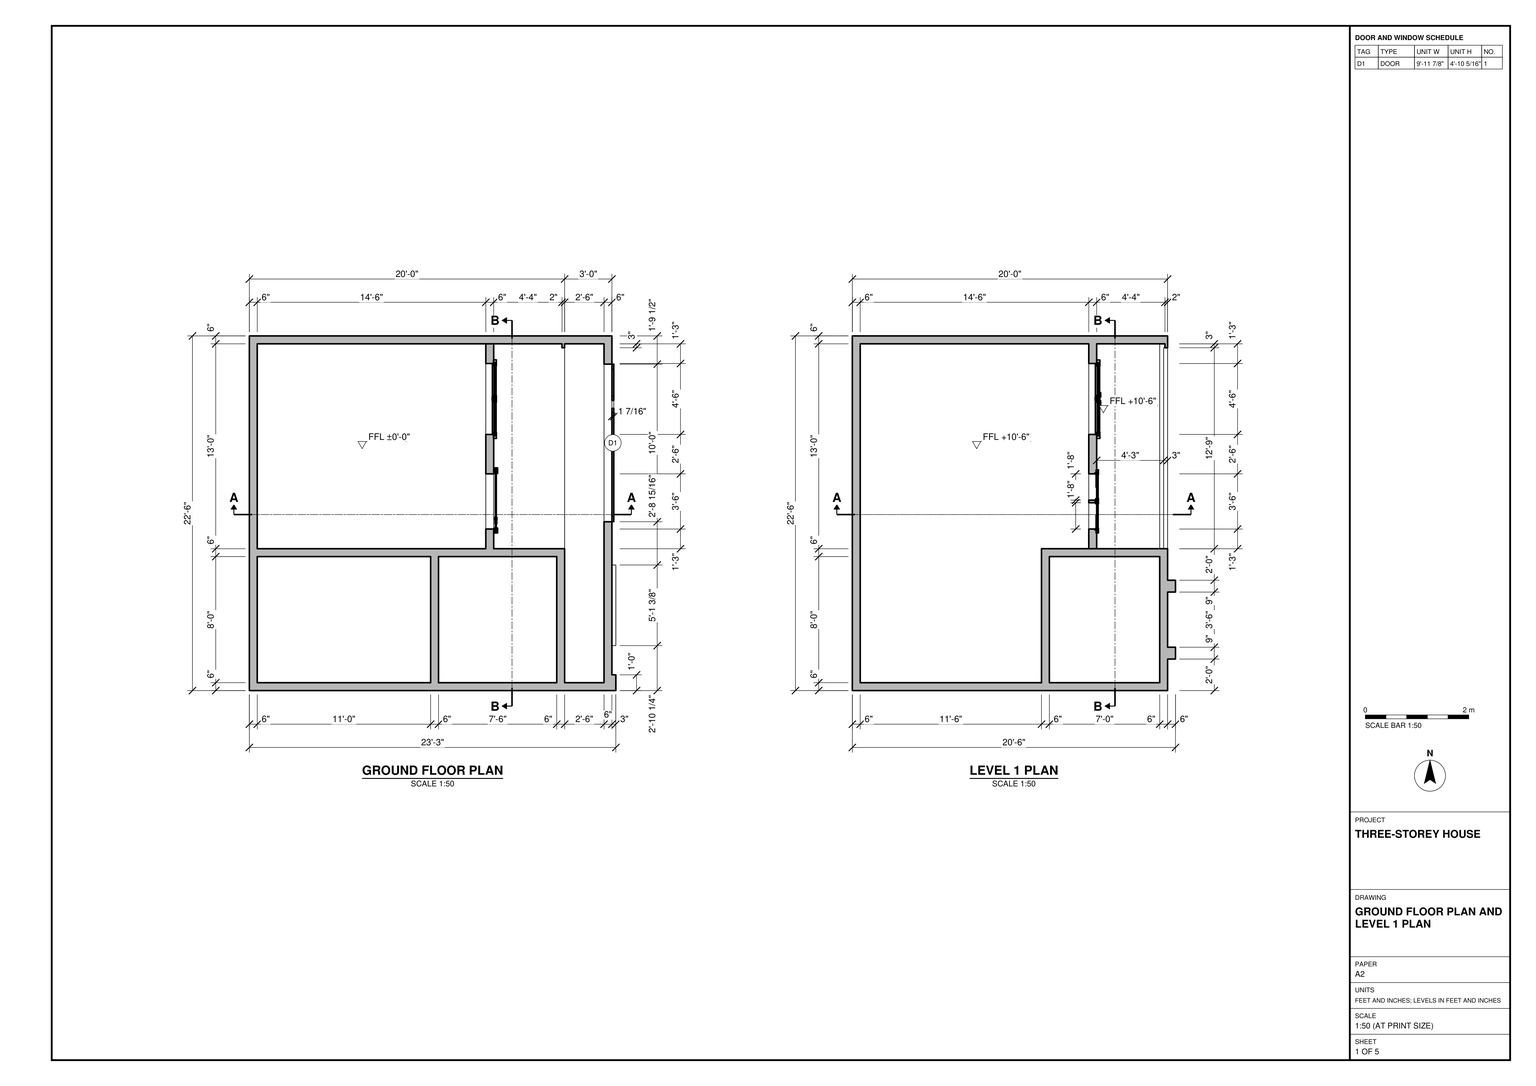
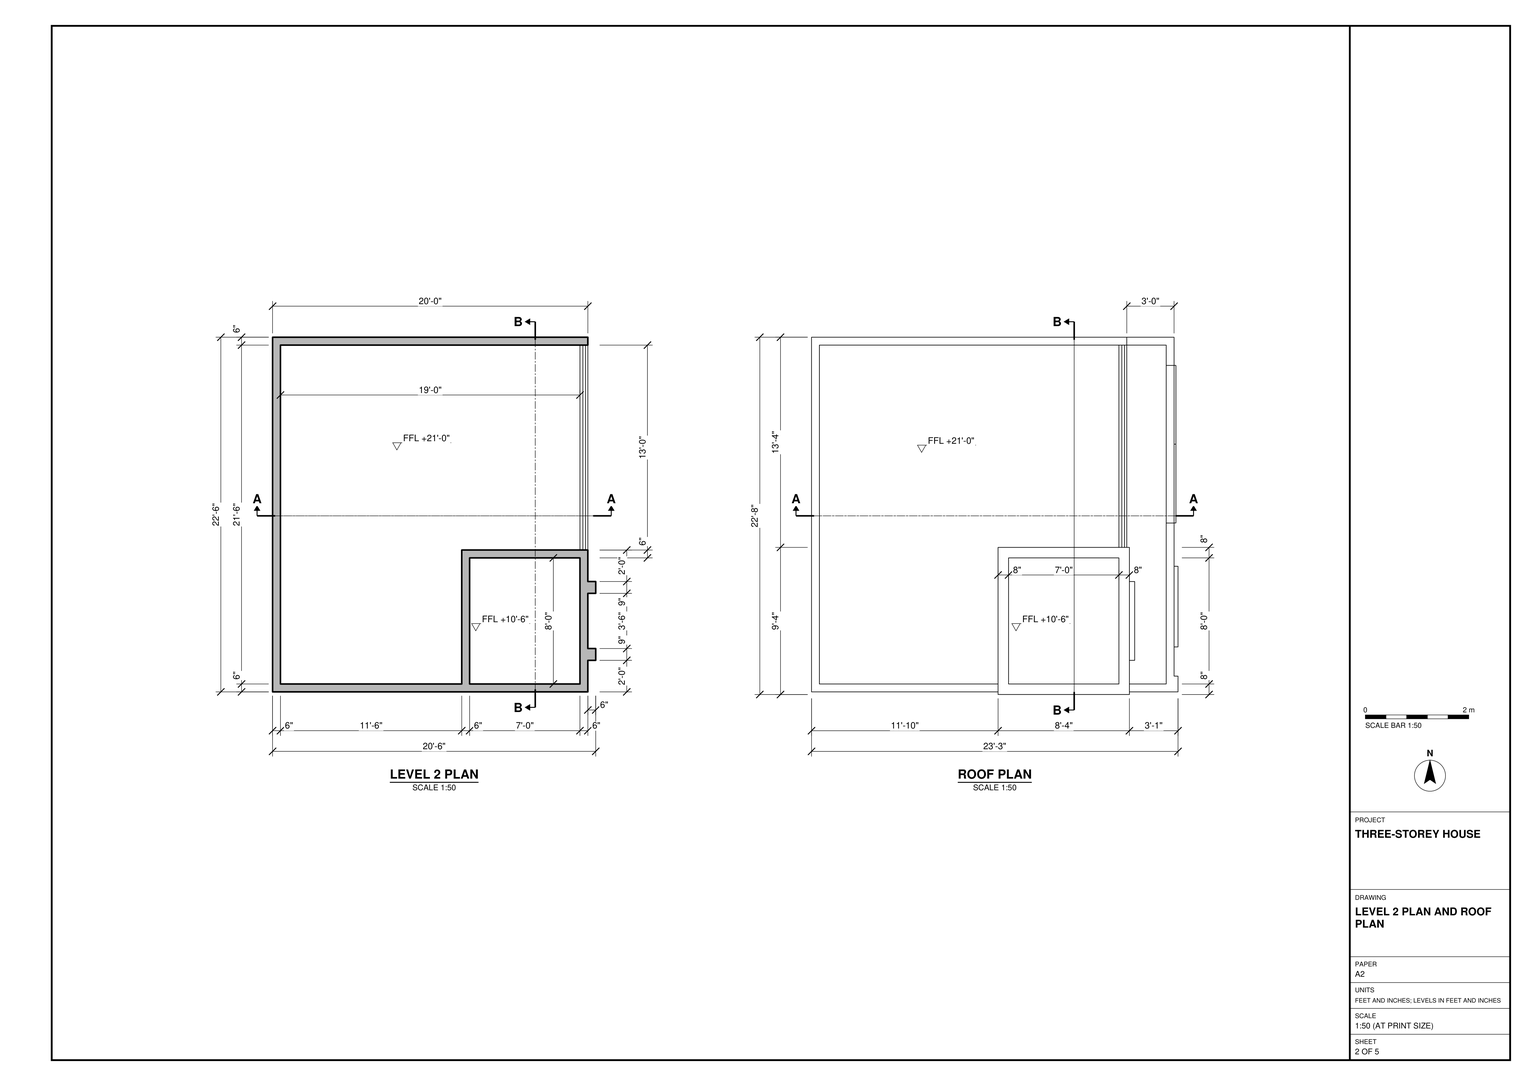
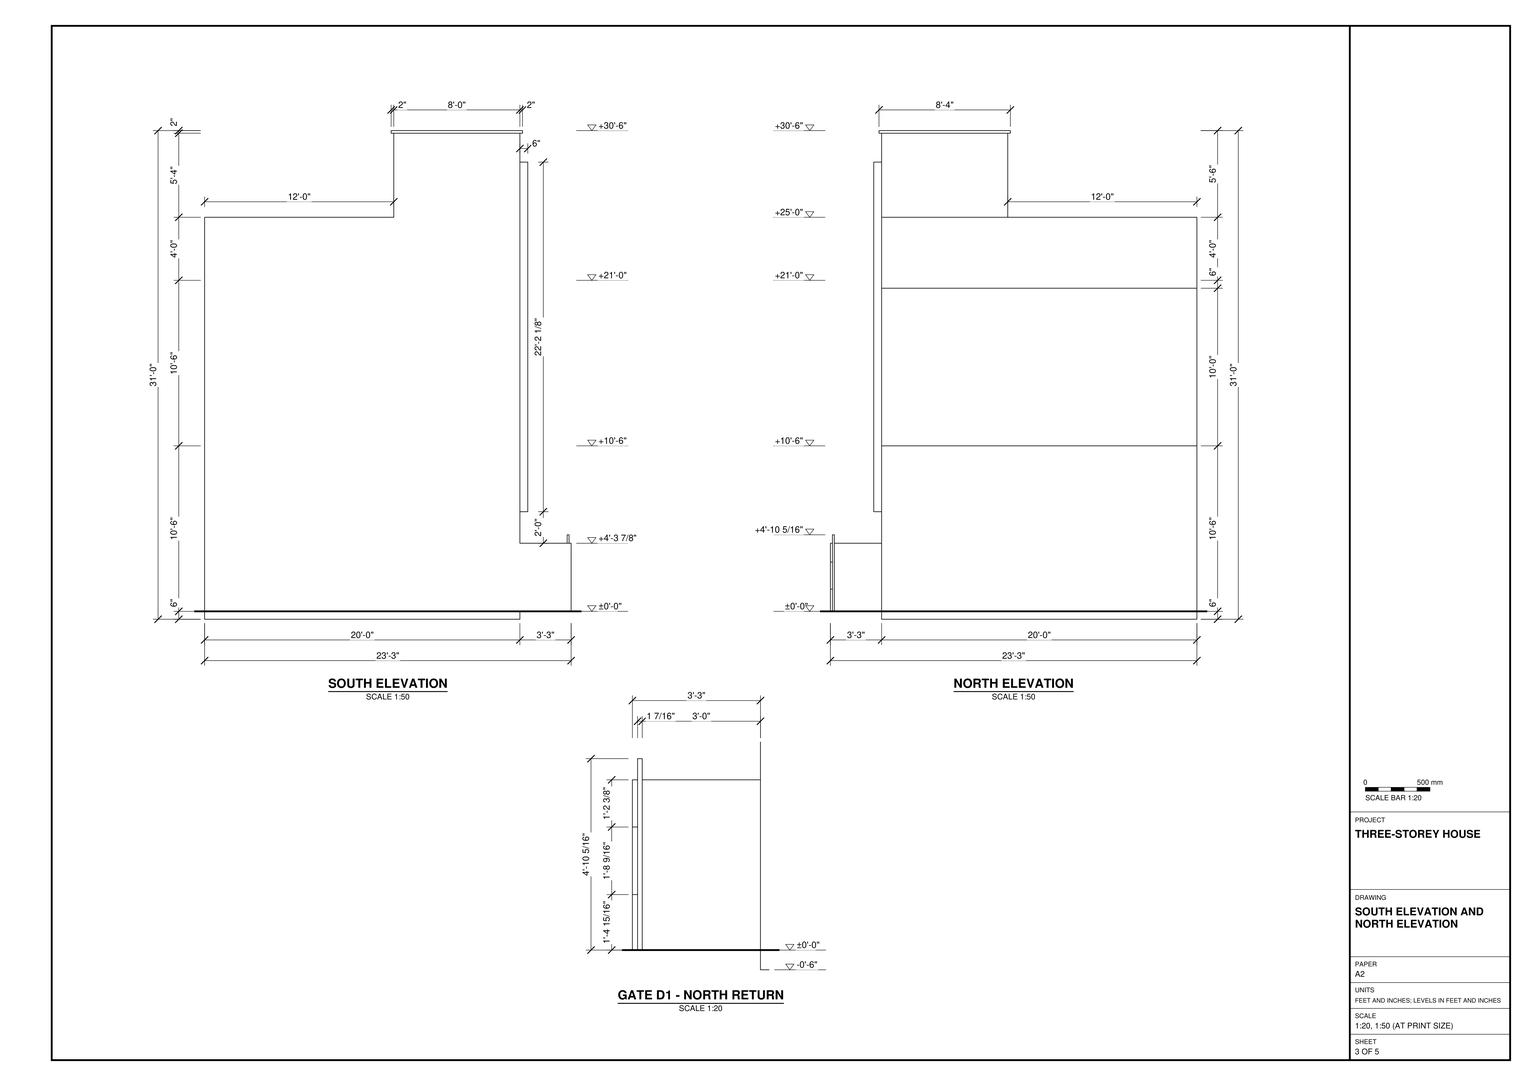
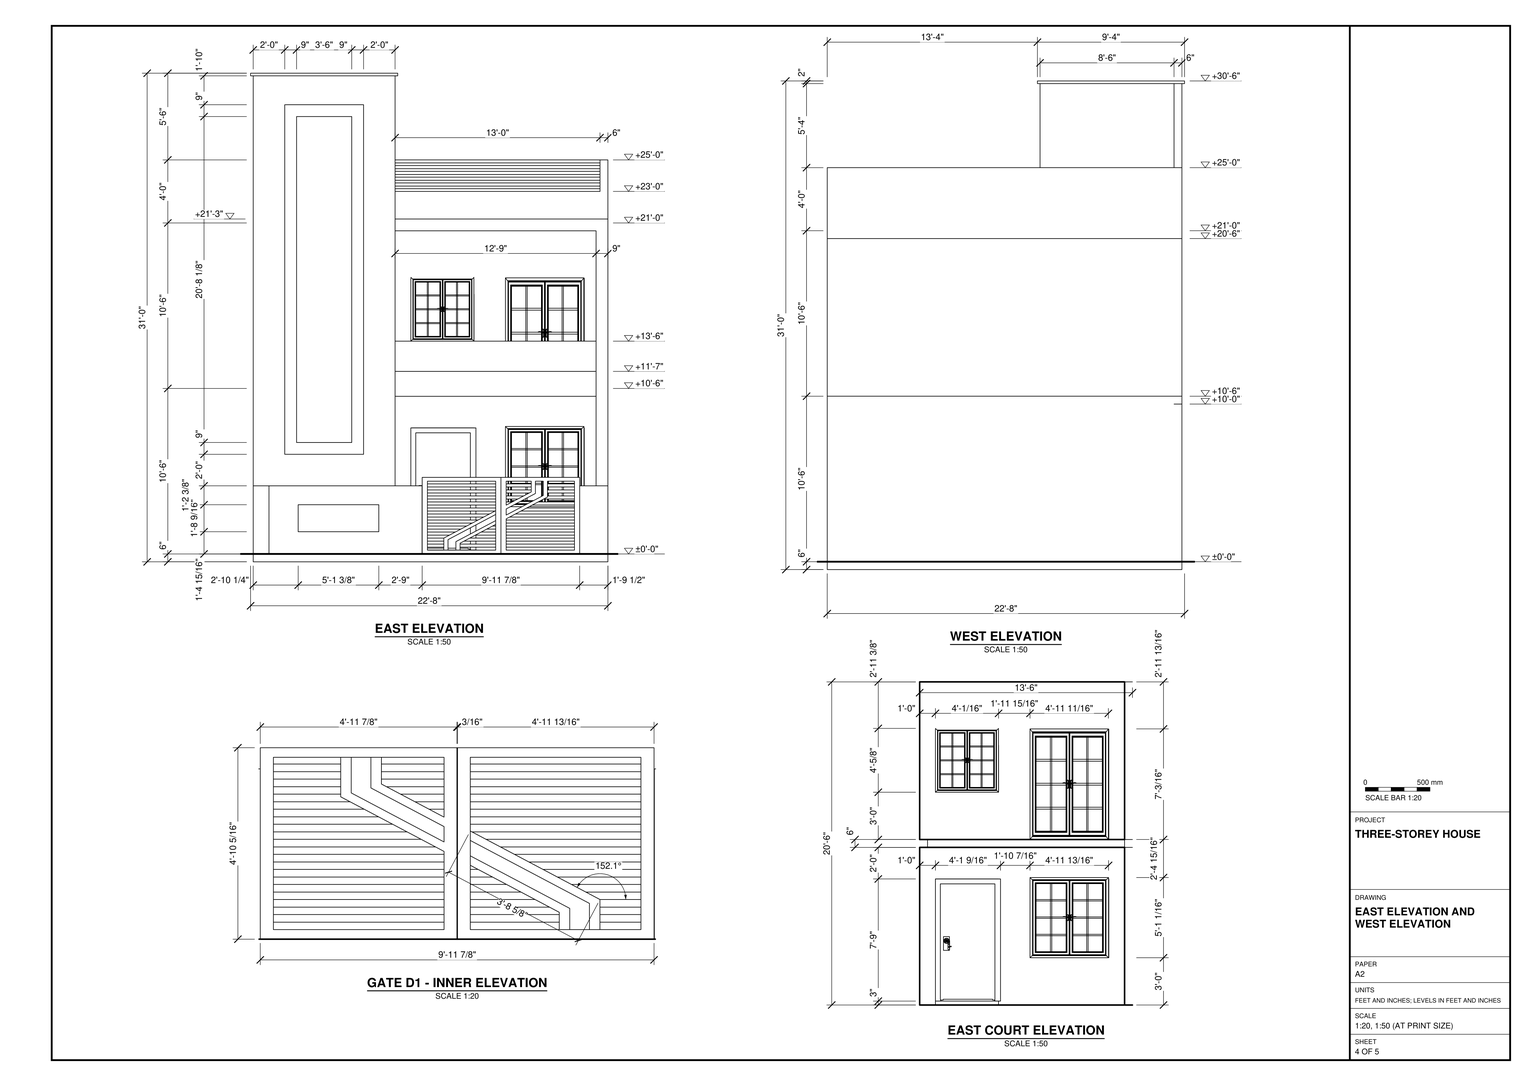
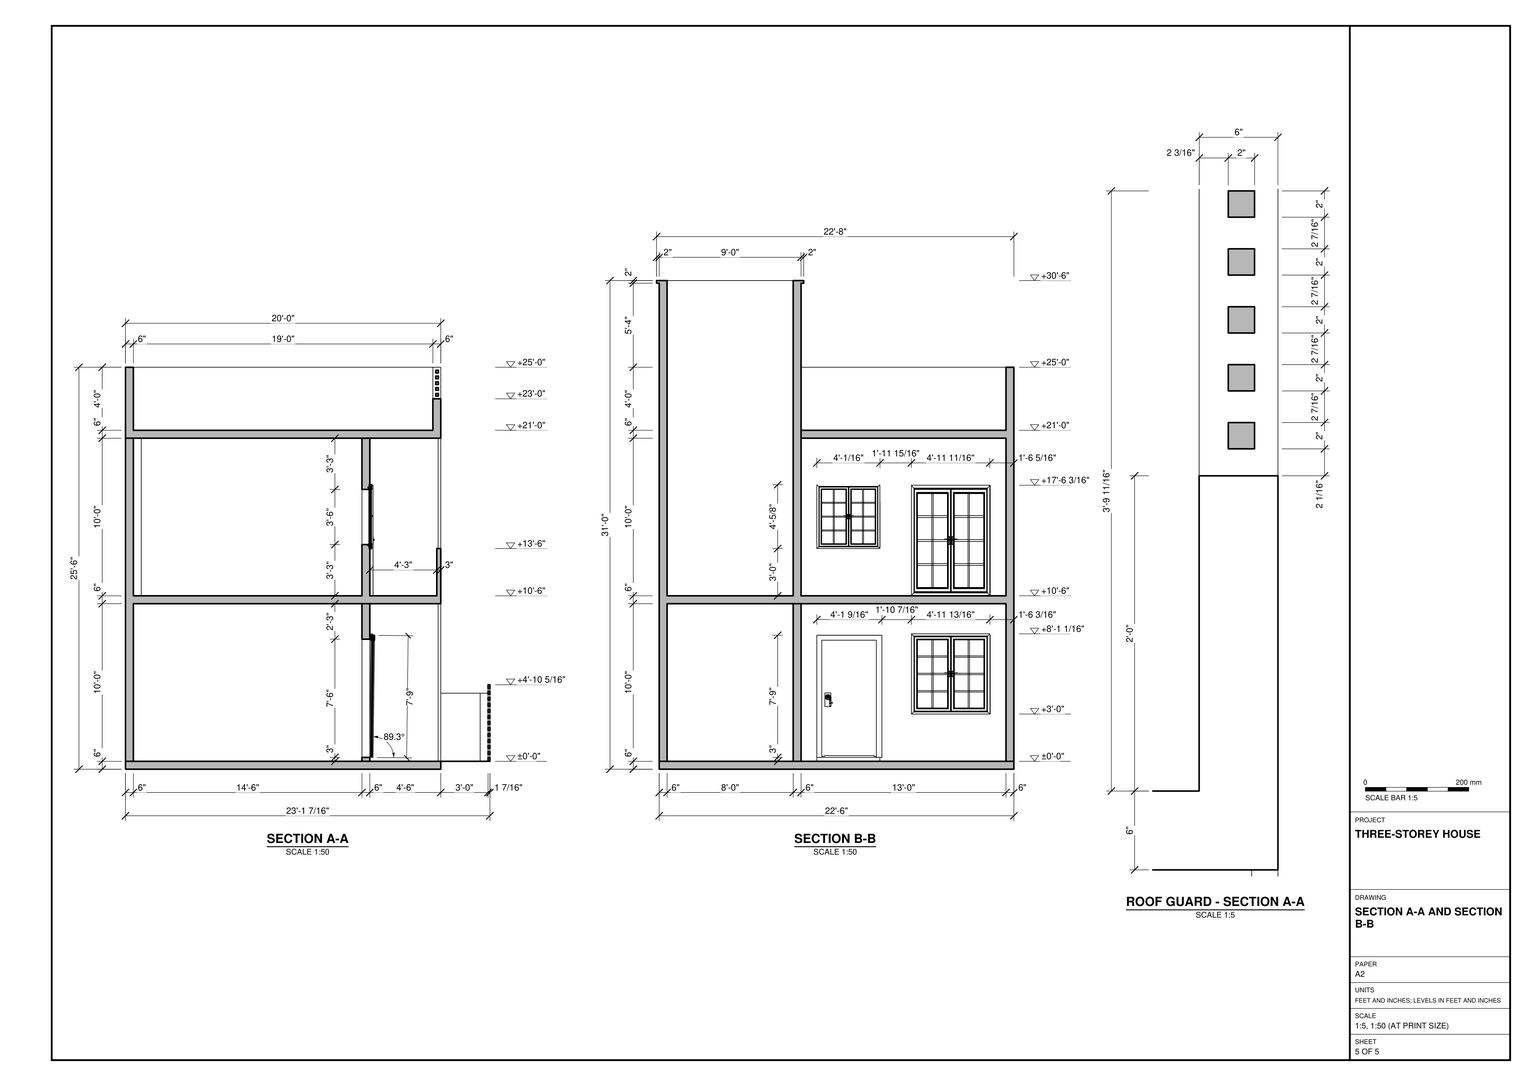
Build the three-storey house in SketchUp from task_files/diagram_01.pdf. Work in feet and inches. Orient the plan with east–west along the x-axis and north–south along the y-axis. The overall extents are 23'-3" along x, 22'-8" along y and 31'-0" vertically. Set the finished floor levels at ±0'-0", +10'-6" and +21'-0".

Start with the ground-floor slab and lay out the walls at their drawn thicknesses. Place the large room in the northwest, the two smaller bays side by side to the south and the narrow access strip along the east edge. Fit the entrance gate in the outer wall of that strip and use the return detail to set its height. Follow the separate upper-floor plans rather than copying the ground-floor partitions upward. Preserve the recessed eastern edge on level 1. At level 2, form the L-shaped terrace around the taller southeast enclosure. Use the elevations to set the parapet heights and the thin projecting cap of the enclosure.

Keep walls, slabs, roof elements and each furniture or joinery piece shown in the drawings in separate groups or components. Use components for repeated parts. Any decor or loose items shown may be suitable library components. Save one SketchUp model as output_files/three_storey_house_with_its_side_gate_and_stepped_roof.skp.

# SketchUp Ruby script. Lengths in inches.
U = 1.inch
M = Sketchup.active_model
def pt(a) = Geom::Point3d.new(a.map { |v| v * U })
def face(e, loops, mat)
  f = e.add_face(loops[0].map { |a| pt(a) })
  loops[1..].each { |l| e.add_face(l.map { |a| pt(a) }).erase! }
  f.material = f.back_material = mat if mat
  f
end
# faces: each face lists its corners as indices into pts; further lists are holes
def faces(e, pts, list, mat = nil) = list.each { |f| face(e, (f[0].is_a?(Array) ? f : [f]).map { |l| l.map { |i| pts[i] } }, mat) }
# xy, xz, yz: faces in a plane at the given z, y or x. An outline is a flat list of corners, or four numbers for a rectangle; further outlines are holes
def ring(l) = l.size == 4 ? [[l[0], l[1]], [l[2], l[1]], [l[2], l[3]], [l[0], l[3]]] : l.each_slice(2).to_a
def flat(e, list, mat, &to3) = list.each { |f| face(e, (f[0].is_a?(Array) ? f : [f]).map { |l| ring(l).map { |u, v| to3.(u, v) } }, mat) }
def xy(e, z, list, mat = nil) = flat(e, list, mat) { |x, y| [x, y, z] }
def xz(e, y, list, mat = nil) = flat(e, list, mat) { |x, z| [x, y, z] }
def yz(e, x, list, mat = nil) = flat(e, list, mat) { |y, z| [x, y, z] }
def lines(e, pts, list) = list.each { |a, b| e.add_line(pt(pts[a]), pt(pts[b])) }
# prism: a flat outline (further loops are holes) pulled along v
def prism(e, loops, v, mat = nil)
  f = face(e, loops, mat); d = Geom::Vector3d.new(v.map { |x| x * U })
  f.pushpull(f.normal.samedirection?(d) ? d.length : -d.length)
end
def box(e, o, s, mat = nil) = prism(e, [[o, [o[0] + s[0], o[1], o[2]], [o[0] + s[0], o[1] + s[1], o[2]], [o[0], o[1] + s[1], o[2]]]], [0, 0, s[2]], mat)
def at(x, y, z, deg = 0) = Geom::Transformation.translation(pt([x, y, z])) * Geom::Transformation.rotation(ORIGIN, Z_AXIS, deg.degrees)
def axes(o, x, y, z) = Geom::Transformation.new([*x, 0, *y, 0, *z, 0, *pt(o).to_a, 1])
def part(name) = M.definitions.add(name)
# library, detail: a bought-in or finely detailed component or shape, given as its bounding box
def library(name, o, s) = part(name).tap { |d| box(d.entities, o, s) }
def detail(e, o, s) = box(e.add_group.entities, o, s)
def put(e, d, t, mat = nil) = e.add_instance(d, t).tap { |i| i.material = mat if mat }
def group(e, t, mat = nil) = e.add_group.tap { |g| g.transformation = t; g.material = mat if mat }.entities
root = M.entities
M.materials.add("B01_Ivory_Dust").color = [255, 217, 206]
M.materials.add("C08_Toffee_Ember").color = [102, 51, 0]
M.materials.add("Glass_Basic_01").color = [161, 173, 186]
M.materials["Glass_Basic_01"].alpha = 0.25
M.materials.add("Marble_01_1K").color = [230, 221, 211]
M.materials.add("Wood_Floor_01_1K").color = [214, 157, 87]
M.materials.add("Wood_Planks_01_1K").color = [69, 67, 63]
M.materials.add("Wood_Veneer_15_1K").color = [103, 69, 45]
c1 = library("porta+4",[0.2,-5.42,1.33],[46.55,4.72,83.21])
c2 = library("Modern+Gate+1",[0,0,0],[118.11,1.97,78.74])
c3 = library("mesh-162",[-1607.75,-1245.64,-53.98],[1739.16,1702.88,120.91])
c4 = part("Group9")
put(c4.entities,c3,at(0,0,0))
xy(root,-6,[[0,2,240,272]])
xy(root,0,[[0,2,240,2,240,110,186,110,186,272,0,272]])
xz(root,2,[[0,-6,240,0]])
xz(root,272,[[0,-6,240,0]])
yz(root,0,[[2,-6,272,0]])
yz(root,240,[[2,-6,272,0]])
g1 = group(root,at(0,2,0))
xy(g1,0,[[0,0,0,102,6,102,6,6,234,6,234,108,240,108,240,0],[138,6,138,102,0,102,0,270,6,270,6,108,180,108,180,264,186,264,186,108,234,108,234,102,144,102,144,6],[6,6,138,102],[144,6,234,102],[238,261,240,264],
  [186,264,240,270]])
xy(g1,0,[[240,0,240,6,270,6,270,128.52,276,128.52,276,12,279,12,279,0],[270,128.52,276,248.52],[270,248.52,270,264,240,264,240,270,276,270,276,248.52]],"B01_Ivory_Dust")
xy(g1,0,[[240,6,270,264],[186,108,186,264,238,264,238,261,240,261,240,108]],"Marble_01_1K")
xy(g1,3,[[180,123,186,165]])
xy(g1,16.91,[[276,34.23,279,95.61]],"Wood_Planks_01_1K")
xy(g1,37.48,[[276,34.23,279,95.61]],"Wood_Planks_01_1K")
xy(g1,39,[[180,195,186,249]])
xy(g1,51.85,[[240,0,279,0,279,12,276,12,276,128.52,270,128.52,270,6,240,6],[270,248.52,276,248.52,276,270,240,270,240,264,270,264]],"B01_Ivory_Dust")
xy(g1,75.85,[[240,24,246,84]],"C08_Toffee_Ember")
xy(g1,84.85,[[240,33,246,75]],"C08_Toffee_Ember")
xy(g1,93,[[180,123,186,165],[180,195,186,249]])
xy(g1,120,[[6,6,138,102],[138,6,144,108],[144,6,234,102],[144,102,234,108],[6,108,180,264],
  [180,108,186,264]])
xy(g1,120,[[186,108,186,264,238,264,238,261,240,261,240,108]],"Wood_Veneer_15_1K")
xy(g1,126,[[6,6,144,6,144,108,180,108,180,264,6,264],[150,6,234,102],[234,108,237,108,237,261,238,261,238,264,234,264]])
xy(g1,126,[[186,108,234,264]],"B01_Ivory_Dust")
xy(g1,129,[[180,195,186,249]])
xy(g1,162,[[237,108,240,261]])
xy(g1,165,[[180,123,186,143],[180,145,186,165]])
xy(g1,207,[[180,123,186,143],[180,145,186,165],[180,195,186,249]])
xy(g1,246,[[0,6,6,108],[6,6,6,264,180,264,180,108,144,108,144,6],[0,108,6,264],[180,108,186,114],[180,114,186,264],
  [0,264,12,270]])
xy(g1,246,[[186,108,186,264,238,264,238,261,240,261,240,108]],"Wood_Veneer_15_1K")
xy(g1,252,[[6,6,144,6,144,108,234,108,234,264,6,264]])
xy(g1,276,[[234,108,240,264]])
xy(g1,278.05,[[236.22,108,238.22,264]])
xy(g1,280.05,[[236.22,108,238.22,264]])
xy(g1,282.46,[[236.22,108,238.22,264]])
xy(g1,284.46,[[236.22,108,238.22,264]])
xy(g1,286.87,[[236.22,108,238.22,264]])
xy(g1,288.87,[[236.22,108,238.22,264]])
xy(g1,291.28,[[236.22,108,238.22,264]])
xy(g1,293.28,[[236.22,108,238.22,264]])
xy(g1,295.6875,[[236.22,108,238.22,264]])
xy(g1,297.6875,[[236.22,108,238.22,264]])
xy(g1,300,[[0,0,144,0,144,6,6,6,6,264,240,264,240,270,0,270]])
xy(g1,333,[[240,33,246,75]],"C08_Toffee_Ember")
xy(g1,342,[[240,24,246,84]],"C08_Toffee_Ember")
xy(g1,364,[[142,-2,240,0],[142,0,144,6],[142,6,144,108],[142,108,240,110]])
xy(g1,364,[[240,-2,242,110]],"C08_Toffee_Ember")
xy(g1,366,[[[142,-2,242,110],[150,6,234,102]]])
xz(g1,-2,[[142,364,242,366]],"C08_Toffee_Ember")
xz(g1,0,[[0,0,279,0,279,51.85,240,51.85,240,364,144,364,144,300,0,300]],"B01_Ivory_Dust")
xz(g1,6,[[6,0,138,104.57],[144,0,234,120],[6,104.57,138,120],[6,120,138,126],[6,126,138,246],
  [138,126,144,246],[150,126,234,366],[6,252,144,300]])
xz(g1,6,[[240,0,270,51.85]],"B01_Ivory_Dust")
xz(g1,12,[[276,0,279,51.85]],"B01_Ivory_Dust")
xz(g1,24,[[240,75.85,246,342]],"C08_Toffee_Ember")
xz(g1,33,[[240,84.85,246,333]],"C08_Toffee_Ember")
xz(g1,34.23,[[276,16.91,279,37.48]],"Wood_Planks_01_1K")
xz(g1,75,[[240,84.85,246,333]],"C08_Toffee_Ember")
xz(g1,84,[[240,75.85,246,342]],"C08_Toffee_Ember")
xz(g1,95.61,[[276,16.91,279,37.48]],"Wood_Planks_01_1K")
xz(g1,102,[[6,0,138,120],[144,0,234,120],[150,126,234,366]])
xz(g1,108,[[6,0,180,120],[144,126,180,246],[180,126,186,246],[237,126,240,162],[144,246,144,252,234,252,234,276,240,276,240,246]])
xz(g1,108,[[186,0,240,120],[186,126,186,246,240,246,240,162,237,162,237,126],[[144,252,144,364,240,364,240,276,234,276,234,252],[236.22,295.6875,238.22,297.6875],[236.22,291.28,238.22,293.28],[236.22,286.87,238.22,288.87],[236.22,282.46,238.22,284.46],[236.22,278.05,238.22,280.05]]],"B01_Ivory_Dust")
xz(g1,110,[[142,364,242,366]],"C08_Toffee_Ember")
xz(g1,123,[[180,3,186,93],[180,165,186,207]])
xz(g1,128.52,[[270,0,276,51.85]],"B01_Ivory_Dust")
xz(g1,143,[[180,165,186,207]])
xz(g1,145,[[180,165,186,207]])
xz(g1,165,[[180,3,186,93],[180,165,186,207]])
xz(g1,195,[[180,39,186,93],[180,129,186,207]])
xz(g1,248.52,[[270,0,276,51.85]],"B01_Ivory_Dust")
xz(g1,249,[[180,39,186,93],[180,129,186,207]])
xz(g1,261,[[237,126,238,162],[238,126,240,162]])
xz(g1,261,[[238,0,240,120],[238,162,240,246]],"Wood_Veneer_15_1K")
xz(g1,264,[[6,0,180,120],[180,0,186,104.57],[180,104.57,186,120],[6,126,12,246],[12,126,180,246],
  [6,252,234,300],[[234,276,240,300],[236.22,278.05,238.22,280.05],[236.22,282.46,238.22,284.46],[236.22,286.87,238.22,288.87],[236.22,291.28,238.22,293.28],[236.22,295.6875,238.22,297.6875]]])
xz(g1,264,[[186,0,238,120],[240,0,270,51.85],[186,126,238,246]],"B01_Ivory_Dust")
xz(g1,270,[[0,0,240,126],[240,0,276,51.85],[0,126,240,246],[0,246,240,300]],"B01_Ivory_Dust")
yz(g1,0,[[0,0,270,126],[0,126,270,246],[0,246,270,300]],"B01_Ivory_Dust")
yz(g1,6,[[6,0,102,104.57],[108,0,264,120],[6,104.57,102,120],[6,126,264,246],[6,252,264,300]])
yz(g1,138,[[6,0,102,104.57],[6,104.57,102,120]])
yz(g1,142,[[-2,364,110,366]],"C08_Toffee_Ember")
yz(g1,144,[[6,0,102,120],[6,126,108,246],[6,246,108,252],[6,252,108,364],[0,300,6,364]])
yz(g1,150,[[6,126,102,366]])
yz(g1,180,[[[108,0,108,120,114,120,114,104.57,264,104.57,264,0],[123,3,165,93],[195,39,249,93]],[114,104.57,264,120],[108,126,114,246],[[114,126,264,246],[195,129,249,207],[145,165,165,207],[123,165,143,207]]])
yz(g1,186,[[[120,0,168,96],[123,3,165,93]],[[192,36,252,96],[195,39,249,93]],[[192,126,252,210],[195,129,249,207]],[[120,162,168,210],[145,165,165,207],[123,165,143,207]]])
yz(g1,186,[[[108,0,120,0,120,96,168,96,168,0,264,0,264,120,108,120],[192,36,252,96]],[[108,126,192,126,192,210,252,210,252,126,264,126,264,246,108,246],[120,162,168,210]]],"B01_Ivory_Dust")
yz(g1,234,[[6,0,102,120],[6,126,102,366],[108,252,264,276]])
yz(g1,236.22,[[108,278.05,264,280.05],[108,282.46,264,284.46],[108,286.87,264,288.87],[108,291.28,264,293.28],[108,295.6875,264,297.6875]])
yz(g1,237,[[108,126,261,162]],"Glass_Basic_01")
yz(g1,238,[[261,0,264,120],[261,126,264,246]])
yz(g1,238.22,[[108,278.05,264,280.05],[108,282.46,264,284.46],[108,286.87,264,288.87],[108,291.28,264,293.28],[108,295.6875,264,297.6875]])
yz(g1,240,[[6,0,108,51.85],[[0,51.85,108,364],[24,75.85,84,342]],[108,120,261,138.99],[108,255,270,255,270,300,264,300,264,276,108,276]],"B01_Ivory_Dust")
yz(g1,240,[[108,138.99,261,162]],"Glass_Basic_01")
yz(g1,240,[[33,84.85,75,333]],"Wood_Floor_01_1K")
yz(g1,240,[[261,0,264,0,264,51.85,270,51.85,270,255,108,255,108,246,261,246]],"Wood_Veneer_15_1K")
yz(g1,242,[[-2,364,110,366]],"C08_Toffee_Ember")
yz(g1,246,[[[24,75.85,84,342],[33,84.85,75,333]]],"C08_Toffee_Ember")
yz(g1,270,[[6,0,128.52,51.85],[248.52,0,264,51.85]],"B01_Ivory_Dust")
yz(g1,276,[[[12,0,128.52,51.85],[34.23,16.91,95.61,37.48]],[248.52,0,270,51.85]],"B01_Ivory_Dust")
yz(g1,279,[[0,0,12,51.85]],"B01_Ivory_Dust")
yz(g1,279,[[34.23,16.91,95.61,37.48]],"Wood_Planks_01_1K")
p = [[234,6,120],[240,6,120],[6,6,120],[0,6,120],[180,114,126],[180,114,120],
  [6,108,104.57],[6,102,104.57],[234,264,126],[234,264,120],[6,264,120],[6,270,120],
  [0,0,120],[6,264,126],[144,0,126],[144,6,126],[144,6,246],[144,0,246],
  [238,264,126],[240,264,126],[238,264,120],[240,264,120]]
lines(g1,p,[[0,1],[2,3],[4,5],[6,7],[8,9],[10,11],[3,12],[10,13],[14,15],[16,17],[18,19],[20,21]])
put(g1,c1,axes([184.16,119.79,1.47],[0,1.06445,0],[-1,0,0],[0,0,1.11822]))
put(g1,c2,axes([277.42,128.62,0],[0,1.0152,0],[-0.72,0,0],[0,0,0.74038]))
put(g1,c4,axes([186.16,132.91,206.92],[0,0,0.02795],[0,-0.02823,0],[0.02795,0,0]))
put(g1,c4,axes([186.54,208.05,92.43],[0,0,0.03511],[0,-0.03511,0],[0.03511,0,0]))
put(g1,c4,axes([186.77,208.02,203.84],[0,0,0.04843],[0,-0.03504,0],[0.03937,0,0]))
